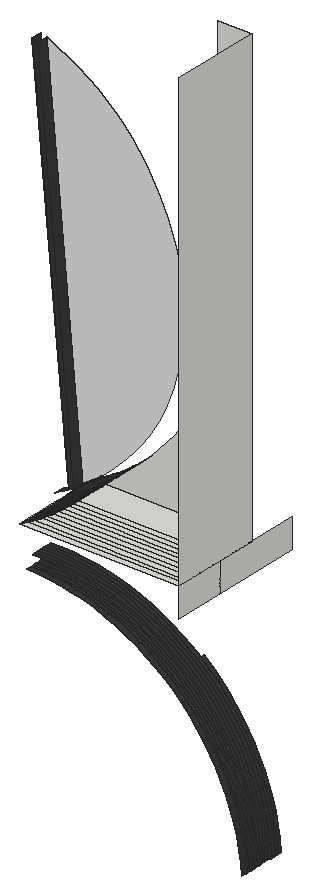
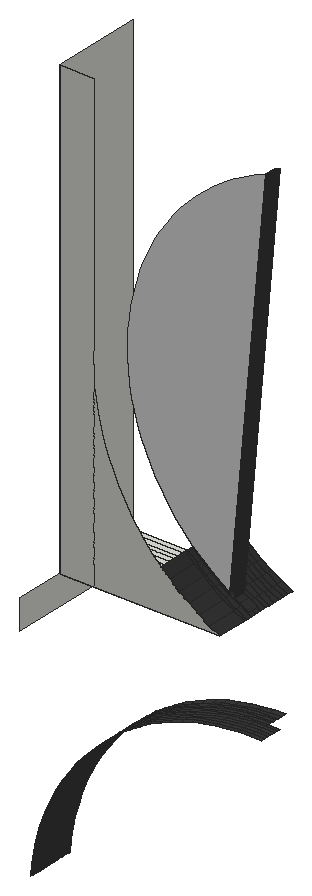
# SketchUp Ruby script. Lengths in inches.
U = 1.inch
M = Sketchup.active_model
def pt(a) = Geom::Point3d.new(a.map { |v| v * U })
def face(e, loops, mat)
  f = e.add_face(loops[0].map { |a| pt(a) })
  loops[1..].each { |l| e.add_face(l.map { |a| pt(a) }).erase! }
  f.material = f.back_material = mat if mat
  f
end
# faces: each face lists its corners as indices into pts; further lists are holes
def faces(e, pts, list, mat = nil) = list.each { |f| face(e, (f[0].is_a?(Array) ? f : [f]).map { |l| l.map { |i| pts[i] } }, mat) }
# xy, xz, yz: faces in a plane at the given z, y or x. An outline is a flat list of corners, or four numbers for a rectangle; further outlines are holes
def ring(l) = l.size == 4 ? [[l[0], l[1]], [l[2], l[1]], [l[2], l[3]], [l[0], l[3]]] : l.each_slice(2).to_a
def flat(e, list, mat, &to3) = list.each { |f| face(e, (f[0].is_a?(Array) ? f : [f]).map { |l| ring(l).map { |u, v| to3.(u, v) } }, mat) }
def xy(e, z, list, mat = nil) = flat(e, list, mat) { |x, y| [x, y, z] }
def xz(e, y, list, mat = nil) = flat(e, list, mat) { |x, z| [x, y, z] }
def yz(e, x, list, mat = nil) = flat(e, list, mat) { |y, z| [x, y, z] }
def lines(e, pts, list) = list.each { |a, b| e.add_line(pt(pts[a]), pt(pts[b])) }
# prism: a flat outline (further loops are holes) pulled along v
def prism(e, loops, v, mat = nil)
  f = face(e, loops, mat); d = Geom::Vector3d.new(v.map { |x| x * U })
  f.pushpull(f.normal.samedirection?(d) ? d.length : -d.length)
end
def box(e, o, s, mat = nil) = prism(e, [[o, [o[0] + s[0], o[1], o[2]], [o[0] + s[0], o[1] + s[1], o[2]], [o[0], o[1] + s[1], o[2]]]], [0, 0, s[2]], mat)
def at(x, y, z, deg = 0) = Geom::Transformation.translation(pt([x, y, z])) * Geom::Transformation.rotation(ORIGIN, Z_AXIS, deg.degrees)
def axes(o, x, y, z) = Geom::Transformation.new([*x, 0, *y, 0, *z, 0, *pt(o).to_a, 1])
def part(name) = M.definitions.add(name)
# library, detail: a bought-in or finely detailed component or shape, given as its bounding box
def library(name, o, s) = part(name).tap { |d| box(d.entities, o, s) }
def detail(e, o, s) = box(e.add_group.entities, o, s)
def put(e, d, t, mat = nil) = e.add_instance(d, t).tap { |i| i.material = mat if mat }
def group(e, t, mat = nil) = e.add_group.tap { |g| g.transformation = t; g.material = mat if mat }.entities
root = M.entities
M.materials.add("[Color M07]").color = [58, 58, 58]
M.materials.add("[Mirror 02]").color = [229, 229, 229]
xy(root,253.6875,[[112.46,0,154.46,1.5],[112.46,1.5,154.46,3],[112.46,3,154.46,4.5],[112.46,4.5,154.46,6],[112.46,6,154.46,7.5],
  [112.46,7.5,154.46,9],[112.46,9,154.46,10.5],[112.46,10.5,154.46,12],[112.46,12,154.46,13.5],[112.46,13.5,154.46,15],
  [112.46,15,154.46,24]])
xz(root,12,[[115.72,257.55,117.05,258.33,107.57,360.4,106.12,360.93]],"[Color M07]")
xz(root,14.875,[[117.05,258.33,119.62,260.05,122.09,261.9,124.46,263.875,126.72,265.98,128.87,268.2,130.89,270.54,132.78,272.98,134.54,275.51,136.16,278.14,137.64,280.85,138.97,283.64,140.15,286.5,141.17,289.41,142.03,292.375,142.74,295.38,143.28,298.42,143.65,301.49,143.87,304.57,143.91,307.66,143.79,310.74,143.51,313.82,143.06,316.87,142.44,319.9,141.67,322.89,140.73,325.83,139.64,328.72,138.39,331.54,137,334.3,135.46,336.97,133.77,339.5625,131.95,342.06,130,344.45,127.93,346.74,125.73,348.91,123.42,350.95,121,352.875,118.49,354.67,115.88,356.32,113.18,357.83,110.41,359.19,107.57,360.4]],"[Mirror 02]")
xz(root,24,[[112.46,253.6875,115.29,255.16,118.03,256.78,120.68,258.55,123.23,260.46,125.68,262.5,128.01,264.68,130.22,266.97,132.31,269.375,134.26,271.89,136.07,274.51,137.75,277.23,139.27,280.02,140.64,282.9,141.86,285.85,142.91,288.85,143.8,291.91,144.53,295.01,145.09,298.15,145.46,301.2,145.46,253.6875],[145.46,253.6875,145.46,301.2,145.47,301.3125,145.69,304.49,145.74,307.68,145.62,310.86,145.46,312.54,145.46,373.6875,154.46,373.6875,154.46,253.6875]])
yz(root,154.46,[[0,246,13.45,253.6875],[13.45,246,37.13,253.6875],[0,253.6875,24,373.6875]])
p = [[160.01,13.45,184.23],[160.01,14.95,184.23],[160.33,14.95,181.21],[160.33,13.45,181.21],[160.01,15.8,184.23],[160.33,15.8,181.21],
  [160.01,16.65,184.23],[160.33,16.65,181.21],[160.01,17.5,184.23],[160.33,17.5,181.21],[160.01,18.35,184.23],[160.33,18.35,181.21],
  [160.01,19.21,184.23],[160.33,19.21,181.21],[160.01,19.95,184.23],[160.33,19.95,181.21],[160.01,21.02,184.23],[160.33,21.02,181.21],
  [160.01,22.08,184.23],[160.33,22.08,181.21],[160.01,23.14,184.23],[160.33,23.14,181.21],[160.01,24.2,184.23],[160.33,24.2,181.21],
  [160.01,25.27,184.23],[160.33,25.27,181.21],[160.01,26.33,184.23],[160.33,26.33,181.21],[159.53,13.45,187.24],[159.53,14.95,187.24],
  [159.53,15.8,187.24],[159.53,16.65,187.24],[159.53,17.5,187.24],[159.53,18.35,187.24],[159.53,19.21,187.24],[159.53,19.95,187.24],
  [159.53,21.02,187.24],[159.53,22.08,187.24],[159.53,23.14,187.24],[159.53,24.2,187.24],[159.53,25.27,187.24],[159.53,26.33,187.24],
  [158.89,13.45,190.21],[158.89,14.95,190.21],[158.89,15.8,190.21],[158.89,16.65,190.21],[158.89,17.5,190.21],[158.89,18.35,190.21],
  [158.89,19.21,190.21],[158.89,19.95,190.21],[158.89,21.02,190.21],[158.89,22.08,190.21],[158.89,23.14,190.21],[158.89,24.2,190.21],
  [158.89,25.27,190.21],[158.89,26.33,190.21],[158.09,13.45,193.15],[158.09,14.95,193.15],[158.09,15.8,193.15],[158.09,16.65,193.15],
  [158.09,17.5,193.15],[158.09,18.35,193.15],[158.09,19.21,193.15],[158.09,19.95,193.15],[158.09,21.02,193.15],[158.09,22.08,193.15],
  [158.09,23.14,193.15],[158.09,24.2,193.15],[158.09,25.27,193.15],[158.09,26.33,193.15],[157.14,13.45,196.03],[157.14,14.95,196.03],
  [157.14,15.8,196.03],[157.14,16.65,196.03],[157.14,17.5,196.03],[157.14,18.35,196.03],[157.14,19.21,196.03],[157.14,19.95,196.03],
  [157.14,21.02,196.03],[157.14,22.08,196.03],[157.14,23.14,196.03],[157.14,24.2,196.03],[157.14,25.27,196.03],[157.14,26.33,196.03],
  [156.04,13.45,198.87],[156.04,14.95,198.87],[156.04,15.8,198.87],[156.04,16.65,198.87],[156.04,17.5,198.87],[156.04,18.35,198.87],
  [156.04,19.21,198.87],[156.04,19.95,198.87],[156.04,21.02,198.87],[156.04,22.08,198.87],[156.04,23.14,198.87],[156.04,24.2,198.87],
  [156.04,25.27,198.87],[156.04,26.33,198.87],[154.78,13.45,201.64],[154.78,14.95,201.64],[154.78,15.8,201.64],[154.78,16.65,201.64],
  [154.78,17.5,201.64],[154.78,18.35,201.64],[154.78,19.21,201.64],[154.78,19.95,201.64],[154.78,21.02,201.64],[154.78,22.08,201.64],
  [154.78,23.14,201.64],[154.78,24.2,201.64],[154.78,25.27,201.64],[154.78,26.33,201.64],[153.38,13.45,204.34],[153.38,14.95,204.34],
  [153.38,15.8,204.34],[153.38,16.65,204.34],[153.38,17.5,204.34],[153.38,18.35,204.34],[153.38,19.21,204.34],[153.38,19.95,204.34],
  [153.38,21.02,204.34],[153.38,22.08,204.34],[153.38,23.14,204.34],[153.38,24.2,204.34],[153.38,25.27,204.34],[153.38,26.33,204.34],
  [151.84,13.45,206.96],[151.84,14.95,206.96],[151.84,15.8,206.96],[151.84,16.65,206.96],[151.84,17.5,206.96],[151.84,18.35,206.96],
  [151.84,19.21,206.96],[151.84,19.95,206.96],[151.84,21.02,206.96],[151.84,22.08,206.96],[151.84,23.14,206.96],[151.84,24.2,206.96],
  [151.84,25.27,206.96],[151.84,26.33,206.96],[150.16,13.45,209.5],[150.16,14.95,209.5],[150.16,15.8,209.5],[150.16,16.65,209.5],
  [150.16,17.5,209.5],[150.16,18.35,209.5],[150.16,19.21,209.5],[150.16,19.95,209.5],[150.16,21.02,209.5],[150.16,22.08,209.5],
  [150.16,23.14,209.5],[150.16,24.2,209.5],[150.16,25.27,209.5],[150.16,26.33,209.5],[148.35,13.45,211.94],[148.35,14.95,211.94],
  [148.35,15.8,211.94],[148.35,16.65,211.94],[148.35,17.5,211.94],[148.35,18.35,211.94],[148.35,19.21,211.94],[148.35,19.95,211.94],
  [148.35,21.02,211.94],[148.35,22.08,211.94],[148.35,23.14,211.94],[148.35,24.2,211.94],[148.35,25.27,211.94],[148.35,26.33,211.94],
  [146.41,13.45,214.29],[146.41,14.95,214.29],[146.41,15.8,214.29],[146.41,16.65,214.29],[146.41,17.5,214.29],[146.41,18.35,214.29],
  [146.41,19.21,214.29],[146.41,19.95,214.29],[146.41,21.02,214.29],[146.41,22.08,214.29],[146.41,23.14,214.29],[146.41,24.2,214.29],
  [146.41,25.27,214.29],[146.41,26.33,214.29],[144.35,13.45,216.52],[144.35,14.95,216.52],[144.35,15.8,216.52],[144.35,16.65,216.52],
  [144.35,17.5,216.52],[144.35,18.35,216.52],[144.35,19.21,216.52],[144.35,19.95,216.52],[144.35,21.02,216.52],[144.35,22.08,216.52],
  [144.35,23.14,216.52],[144.35,24.2,216.52],[144.35,25.27,216.52],[144.35,26.33,216.52],[142.17,13.45,218.65],[142.17,14.95,218.65],
  [142.17,15.8,218.65],[142.17,16.65,218.65],[142.17,17.5,218.65],[142.17,18.35,218.65],[142.17,19.21,218.65],[142.17,19.95,218.65],
  [142.17,21.02,218.65],[142.17,22.08,218.65],[142.17,23.14,218.65],[142.17,24.2,218.65],[142.17,25.27,218.65],[142.17,26.33,218.65],
  [139.88,13.45,220.65],[139.88,14.95,220.65],[139.88,15.8,220.65],[139.88,16.65,220.65],[139.88,17.5,220.65],[139.88,18.35,220.65],
  [139.88,19.21,220.65],[139.88,19.95,220.65],[139.88,21.02,220.65],[139.88,22.08,220.65],[139.88,23.14,220.65],[139.88,24.2,220.65],
  [139.88,25.27,220.65],[139.88,26.33,220.65],[137.49,13.45,222.53],[137.49,14.95,222.53],[137.49,15.8,222.53],[137.49,16.65,222.53],
  [137.49,17.5,222.53],[137.49,18.35,222.53],[137.49,19.21,222.53],[137.49,19.95,222.53],[137.49,21.02,222.53],[137.49,22.08,222.53],
  [137.49,23.14,222.53],[137.49,24.2,222.53],[137.49,25.27,222.53],[135,13.45,224.28],[135,14.95,224.28],[135,15.8,224.28],
  [135,16.65,224.28],[135,17.5,224.28],[135,18.35,224.28],[135,19.21,224.28],[135,19.95,224.28],[135,21.02,224.28],
  [135,22.08,224.28],[135,23.14,224.28],[135,24.2,224.28],[135,25.27,224.28],[132.42,13.45,225.9],[132.42,14.95,225.9],
  [132.42,15.8,225.9],[132.42,16.65,225.9],[132.42,17.5,225.9],[132.42,18.35,225.9],[132.42,19.21,225.9],[132.42,19.95,225.9],
  [132.42,21.02,225.9],[132.42,22.08,225.9],[132.42,23.14,225.9],[132.42,24.2,225.9],[132.42,25.27,225.9],[129.76,13.45,227.37],
  [129.76,14.95,227.37],[129.76,15.8,227.37],[129.76,16.65,227.37],[129.76,17.5,227.37],[129.76,18.35,227.37],[129.76,19.21,227.37],
  [129.76,19.95,227.37],[129.76,21.02,227.37],[129.76,22.08,227.37],[129.76,23.14,227.37],[129.76,24.2,227.37],[129.76,25.27,227.37],
  [127.02,13.45,228.7],[127.02,14.95,228.7],[127.02,15.8,228.7],[127.02,16.65,228.7],[127.02,17.5,228.7],[127.02,18.35,228.7],
  [127.02,19.21,228.7],[127.02,19.95,228.7],[127.02,21.02,228.7],[127.02,22.08,228.7],[127.02,23.14,228.7],[127.02,24.2,228.7],
  [127.02,25.27,228.7],[124.22,13.45,229.89],[124.22,14.95,229.89],[124.22,15.8,229.89],[124.22,16.65,229.89],[124.22,17.5,229.89],
  [124.22,18.35,229.89],[124.22,19.21,229.89],[124.22,19.95,229.89],[124.22,21.02,229.89],[124.22,22.08,229.89],[124.22,23.14,229.89],
  [124.22,24.2,229.89],[124.22,25.27,229.89],[121.36,13.45,230.92],[121.36,14.95,230.92],[121.36,15.8,230.92],[121.36,16.65,230.92],
  [121.36,17.5,230.92],[121.36,18.35,230.92],[121.36,19.21,230.92],[121.36,19.95,230.92],[121.36,21.02,230.92],[121.36,22.08,230.92],
  [121.36,23.14,230.92],[121.36,24.2,230.92],[121.36,25.27,230.92],[118.45,13.45,231.8],[118.45,14.95,231.8],[118.45,15.8,231.8],
  [118.45,16.65,231.8],[118.45,17.5,231.8],[118.45,18.35,231.8],[118.45,19.21,231.8],[118.45,19.95,231.8],[118.45,21.02,231.8],
  [118.45,22.08,231.8],[118.45,23.14,231.8],[118.45,24.2,231.8],[118.45,25.27,231.8],[115.49,13.45,232.52],[115.49,14.95,232.52],
  [115.49,15.8,232.52],[115.49,16.65,232.52],[115.49,17.5,232.52],[115.49,18.35,232.52],[115.49,19.21,232.52],[115.49,19.95,232.52],
  [115.49,21.02,232.52],[115.49,22.08,232.52],[115.49,23.14,232.52],[115.49,24.2,232.52],[115.49,25.27,232.52],[112.5,13.45,233.08],
  [112.5,14.95,233.08],[112.5,15.8,233.08],[112.5,16.65,233.08],[112.5,17.5,233.08],[112.5,18.35,233.08],[112.5,19.21,233.08],
  [112.5,19.95,233.08],[112.5,21.02,233.08],[112.5,22.08,233.08],[112.5,23.14,233.08],[112.5,24.2,233.08],[112.5,25.27,233.08],
  [109.49,13.45,233.49],[109.49,14.95,233.49],[109.49,15.8,233.49],[109.49,16.65,233.49],[109.49,17.5,233.49],[109.49,18.35,233.49],
  [109.49,19.21,233.49],[109.49,19.95,233.49],[109.49,21.02,233.49],[109.49,22.08,233.49],[109.49,23.14,233.49],[109.49,24.2,233.49],
  [109.49,25.27,233.49],[106.46,13.45,233.73],[106.46,14.95,233.73],[106.46,15.8,233.73],[106.46,16.65,233.73],[106.46,17.5,233.73],
  [106.46,18.35,233.73],[106.46,19.21,233.73],[106.46,19.95,233.73],[106.46,21.02,233.73],[106.46,22.08,233.73],[106.46,23.14,233.73],
  [106.46,24.2,233.73],[106.46,25.27,233.73],[103.41,13.45,233.8125],[103.41,14.95,233.8125],[103.41,15.8,233.8125],[103.41,16.65,233.8125],
  [103.41,17.5,233.8125],[103.41,18.35,233.8125],[103.41,19.21,233.8125],[100.375,19.21,233.73],[100.375,19.95,233.73],[103.41,19.95,233.8125],
  [100.375,21.02,233.73],[103.41,21.02,233.8125],[100.375,22.08,233.73],[103.41,22.08,233.8125],[100.375,23.14,233.73],[103.41,23.14,233.8125],
  [100.375,24.2,233.73],[103.41,24.2,233.8125],[100.375,25.27,233.73],[103.41,25.27,233.8125],[115.29,0,255.16],[115.29,1.5,255.16],
  [112.46,1.5,253.6875],[112.46,0,253.6875],[115.29,3,255.16],[112.46,3,253.6875],[115.29,4.5,255.16],[112.46,4.5,253.6875],
  [115.29,6,255.16],[112.46,6,253.6875],[115.29,7.5,255.16],[112.46,7.5,253.6875],[115.29,9,255.16],[112.46,9,253.6875],
  [115.29,10.5,255.16],[112.46,10.5,253.6875],[115.29,12,255.16],[112.46,12,253.6875],[115.29,13.5,255.16],[112.46,13.5,253.6875],
  [115.29,15,255.16],[112.46,15,253.6875],[115.29,15.8125,255.16],[112.46,15.8125,253.6875],[112.46,24,253.6875],[115.29,24,255.16],
  [118.03,0,256.78],[118.03,1.5,256.78],[118.03,3,256.78],[118.03,4.5,256.78],[118.03,6,256.78],[118.03,7.5,256.78],
  [118.03,9,256.78],[118.03,10.5,256.78],[118.03,12,256.78],[118.03,13.5,256.78],[118.03,15,256.78],[118.03,15.8125,256.78],
  [118.03,24,256.78],[114.4,14.875,256.76],[112.01,14.875,255.52],[112.01,12,255.52],[114.4,12,256.76],[120.68,0,258.55],
  [120.68,1.5,258.55],[120.68,3,258.55],[120.68,4.5,258.55],[120.68,6,258.55],[120.68,7.5,258.55],[120.68,9,258.55],
  [120.68,10.5,258.55],[120.68,12,258.55],[115.72,14.875,257.55],[115.72,12,257.55],[120.68,13.5,258.55],[120.68,15,258.55],
  [120.68,15.8125,258.55],[120.68,24,258.55],[106.12,14.875,360.93],[106.12,12,360.93],[117.05,14.875,258.33],[107.57,14.875,360.4],
  [107.57,12,360.4],[117.05,12,258.33],[119.62,14.875,260.05],[119.62,12,260.05],[123.23,0,260.46],[123.23,1.5,260.46],
  [123.23,3,260.46],[123.23,4.5,260.46],[123.23,6,260.46],[123.23,7.5,260.46],[123.23,9,260.46],[123.23,10.5,260.46],
  [123.23,12,260.46],[123.23,13.5,260.46],[123.23,15,260.46],[123.23,15.8125,260.46],[123.23,24,260.46],[122.09,14.875,261.9],
  [122.09,12,261.9],[125.68,0,262.5],[125.68,1.5,262.5],[125.68,3,262.5],[125.68,4.5,262.5],[125.68,6,262.5],
  [125.68,7.5,262.5],[125.68,9,262.5],[125.68,10.5,262.5],[125.68,12,262.5],[125.68,13.5,262.5],[125.68,15,262.5],
  [125.68,15.8125,262.5],[125.68,24,262.5],[124.46,14.875,263.875],[124.46,12,263.875],[128.01,0,264.68],[128.01,1.5,264.68],
  [128.01,3,264.68],[128.01,4.5,264.68],[128.01,6,264.68],[128.01,7.5,264.68],[128.01,9,264.68],[128.01,10.5,264.68],
  [128.01,12,264.68],[128.01,13.5,264.68],[128.01,15,264.68],[128.01,15.8125,264.68],[128.01,24,264.68]]
faces(root,p,[[0,1,2,3],[1,4,5,2],[4,6,7,5],[6,8,9,7],[8,10,11,9],[10,12,13,11],[12,14,15,13],[14,16,17,15],
  [16,18,19,17],[18,20,21,19],[20,22,23,21],[22,24,25,23],[24,26,27,25],[28,29,1,0],[29,30,4,1],[30,31,6,4],
  [31,32,8,6],[32,33,10,8],[33,34,12,10],[34,35,14,12],[35,36,16,14],[36,37,18,16],[37,38,20,18],[38,39,22,20],
  [39,40,24,22],[40,41,26,24],[42,43,29,28],[43,44,30,29],[44,45,31,30],[45,46,32,31],[46,47,33,32],[47,48,34,33],
  [48,49,35,34],[49,50,36,35],[50,51,37,36],[51,52,38,37],[52,53,39,38],[53,54,40,39],[54,55,41,40],[56,57,43,42],
  [57,58,44,43],[58,59,45,44],[59,60,46,45],[60,61,47,46],[61,62,48,47],[62,63,49,48],[63,64,50,49],[64,65,51,50],
  [65,66,52,51],[66,67,53,52],[67,68,54,53],[68,69,55,54],[70,71,57,56],[71,72,58,57],[72,73,59,58],[73,74,60,59],
  [74,75,61,60],[75,76,62,61],[76,77,63,62],[77,78,64,63],[78,79,65,64],[79,80,66,65],[80,81,67,66],[81,82,68,67],
  [82,83,69,68],[84,85,71,70],[85,86,72,71],[86,87,73,72],[87,88,74,73],[88,89,75,74],[89,90,76,75],[90,91,77,76],
  [91,92,78,77],[92,93,79,78],[93,94,80,79],[94,95,81,80],[95,96,82,81],[96,97,83,82],[98,99,85,84],[99,100,86,85],
  [100,101,87,86],[101,102,88,87],[102,103,89,88],[103,104,90,89],[104,105,91,90],[105,106,92,91],[106,107,93,92],[107,108,94,93],
  [108,109,95,94],[109,110,96,95],[110,111,97,96],[112,113,99,98],[113,114,100,99],[114,115,101,100],[115,116,102,101],[116,117,103,102],
  [117,118,104,103],[118,119,105,104],[119,120,106,105],[120,121,107,106],[121,122,108,107],[122,123,109,108],[123,124,110,109],[124,125,111,110],
  [126,127,113,112],[127,128,114,113],[128,129,115,114],[129,130,116,115],[130,131,117,116],[131,132,118,117],[132,133,119,118],[133,134,120,119],
  [134,135,121,120],[135,136,122,121],[136,137,123,122],[137,138,124,123],[138,139,125,124],[140,141,127,126],[141,142,128,127],[142,143,129,128],
  [143,144,130,129],[144,145,131,130],[145,146,132,131],[146,147,133,132],[147,148,134,133],[148,149,135,134],[149,150,136,135],[150,151,137,136],
  [151,152,138,137],[152,153,139,138],[154,155,141,140],[155,156,142,141],[156,157,143,142],[157,158,144,143],[158,159,145,144],[159,160,146,145],
  [160,161,147,146],[161,162,148,147],[162,163,149,148],[163,164,150,149],[164,165,151,150],[165,166,152,151],[166,167,153,152],[168,169,155,154],
  [169,170,156,155],[170,171,157,156],[171,172,158,157],[172,173,159,158],[173,174,160,159],[174,175,161,160],[175,176,162,161],[176,177,163,162],
  [177,178,164,163],[178,179,165,164],[179,180,166,165],[180,181,167,166],[182,183,169,168],[183,184,170,169],[184,185,171,170],[185,186,172,171],
  [186,187,173,172],[187,188,174,173],[188,189,175,174],[189,190,176,175],[190,191,177,176],[191,192,178,177],[192,193,179,178],[193,194,180,179],
  [194,195,181,180],[196,197,183,182],[197,198,184,183],[198,199,185,184],[199,200,186,185],[200,201,187,186],[201,202,188,187],[202,203,189,188],
  [203,204,190,189],[204,205,191,190],[205,206,192,191],[206,207,193,192],[207,208,194,193],[208,209,195,194],[210,211,197,196],[211,212,198,197],
  [212,213,199,198],[213,214,200,199],[214,215,201,200],[215,216,202,201],[216,217,203,202],[217,218,204,203],[218,219,205,204],[219,220,206,205],
  [220,221,207,206],[221,222,208,207],[222,223,209,208],[224,225,211,210],[225,226,212,211],[226,227,213,212],[227,228,214,213],[228,229,215,214],
  [229,230,216,215],[230,231,217,216],[231,232,218,217],[232,233,219,218],[233,234,220,219],[234,235,221,220],[235,236,222,221],[237,238,225,224],
  [238,239,226,225],[239,240,227,226],[240,241,228,227],[241,242,229,228],[242,243,230,229],[243,244,231,230],[244,245,232,231],[245,246,233,232],
  [246,247,234,233],[247,248,235,234],[248,249,236,235],[250,251,238,237],[251,252,239,238],[252,253,240,239],[253,254,241,240],[254,255,242,241],
  [255,256,243,242],[256,257,244,243],[257,258,245,244],[258,259,246,245],[259,260,247,246],[260,261,248,247],[261,262,249,248],[263,264,251,250],
  [264,265,252,251],[265,266,253,252],[266,267,254,253],[267,268,255,254],[268,269,256,255],[269,270,257,256],[270,271,258,257],[271,272,259,258],
  [272,273,260,259],[273,274,261,260],[274,275,262,261],[276,277,264,263],[277,278,265,264],[278,279,266,265],[279,280,267,266],[280,281,268,267],
  [281,282,269,268],[282,283,270,269],[283,284,271,270],[284,285,272,271],[285,286,273,272],[286,287,274,273],[287,288,275,274],[289,290,277,276],
  [290,291,278,277],[291,292,279,278],[292,293,280,279],[293,294,281,280],[294,295,282,281],[295,296,283,282],[296,297,284,283],[297,298,285,284],
  [298,299,286,285],[299,300,287,286],[300,301,288,287],[302,303,290,289],[303,304,291,290],[304,305,292,291],[305,306,293,292],[306,307,294,293],
  [307,308,295,294],[308,309,296,295],[309,310,297,296],[310,311,298,297],[311,312,299,298],[312,313,300,299],[313,314,301,300],[315,316,303,302],
  [316,317,304,303],[317,318,305,304],[318,319,306,305],[319,320,307,306],[320,321,308,307],[321,322,309,308],[322,323,310,309],[323,324,311,310],
  [324,325,312,311],[325,326,313,312],[326,327,314,313],[328,329,316,315],[329,330,317,316],[330,331,318,317],[331,332,319,318],[332,333,320,319],
  [333,334,321,320],[334,335,322,321],[335,336,323,322],[336,337,324,323],[337,338,325,324],[338,339,326,325],[339,340,327,326],[341,342,329,328],
  [342,343,330,329],[343,344,331,330],[344,345,332,331],[345,346,333,332],[346,347,334,333],[347,348,335,334],[348,349,336,335],[349,350,337,336],
  [350,351,338,337],[351,352,339,338],[352,353,340,339],[354,355,342,341],[355,356,343,342],[356,357,344,343],[357,358,345,344],[358,359,346,345],
  [359,360,347,346],[360,361,348,347],[361,362,349,348],[362,363,350,349],[363,364,351,350],[364,365,352,351],[365,366,353,352],[367,368,355,354],
  [368,369,356,355],[369,370,357,356],[370,371,358,357],[371,372,359,358],[372,373,360,359],[373,374,361,360],[374,375,362,361],[375,376,363,362],
  [376,377,364,363],[377,378,365,364],[378,379,366,365],[380,381,368,367],[381,382,369,368],[382,383,370,369],[383,384,371,370],[384,385,372,371],
  [385,386,373,372],[387,388,389,386],[386,389,374,373],[388,390,391,389],[389,391,375,374],[390,392,393,391],[391,393,376,375],[392,394,395,393],
  [393,395,377,376],[394,396,397,395],[395,397,378,377],[396,398,399,397],[397,399,379,378],[400,401,402,403],[401,404,405,402],[404,406,407,405],
  [406,408,409,407],[408,410,411,409],[410,412,413,411],[412,414,415,413],[414,416,417,415],[418,416,417,419],[420,418,419,421],[422,423,421,420],
  [424,423,422,425],[426,427,401,400],[427,428,404,401],[428,429,406,404],[429,430,408,406],[430,431,410,408],[431,432,412,410],[432,433,414,412],
  [433,434,416,414],[435,434,416,418],[436,435,418,420],[437,422,420,436],[425,422,437,438],[439,440,441,442],[443,444,427,426],[444,445,428,427],
  [445,446,429,428],[446,447,430,429],[447,448,431,430],[448,449,432,431],[449,450,433,432],[450,451,434,433],[452,439,442,453],[454,451,434,435],
  [455,454,435,436],[456,437,436,455],[438,437,456,457],[458,452,453,459],[460,461,462,463],[464,460,463,465],[466,467,444,443],[467,468,445,444],
  [468,469,446,445],[469,470,447,446],[470,471,448,447],[471,472,449,448],[472,473,450,449],[473,474,451,450],[475,474,451,454],[476,475,454,455],
  [477,456,455,476],[457,456,477,478],[479,464,465,480],[481,482,467,466],[482,483,468,467],[483,484,469,468],[484,485,470,469],[485,486,471,470],
  [486,487,472,471],[487,488,473,472],[488,489,474,473],[490,489,474,475],[491,490,475,476],[492,477,476,491],[478,477,492,493],[494,479,480,495],
  [496,497,482,481],[497,498,483,482],[498,499,484,483],[499,500,485,484],[500,501,486,485],[501,502,487,486],[502,503,488,487],[503,504,489,488],
  [505,504,489,490],[506,505,490,491],[507,492,491,506],[493,492,507,508]],"[Color M07]")
